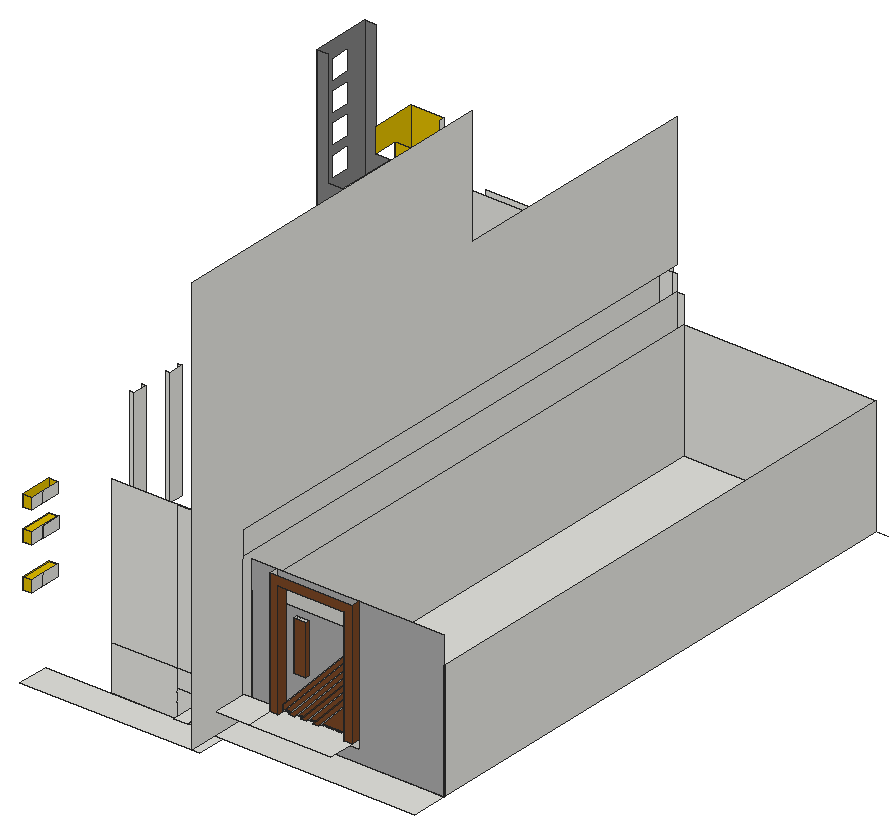
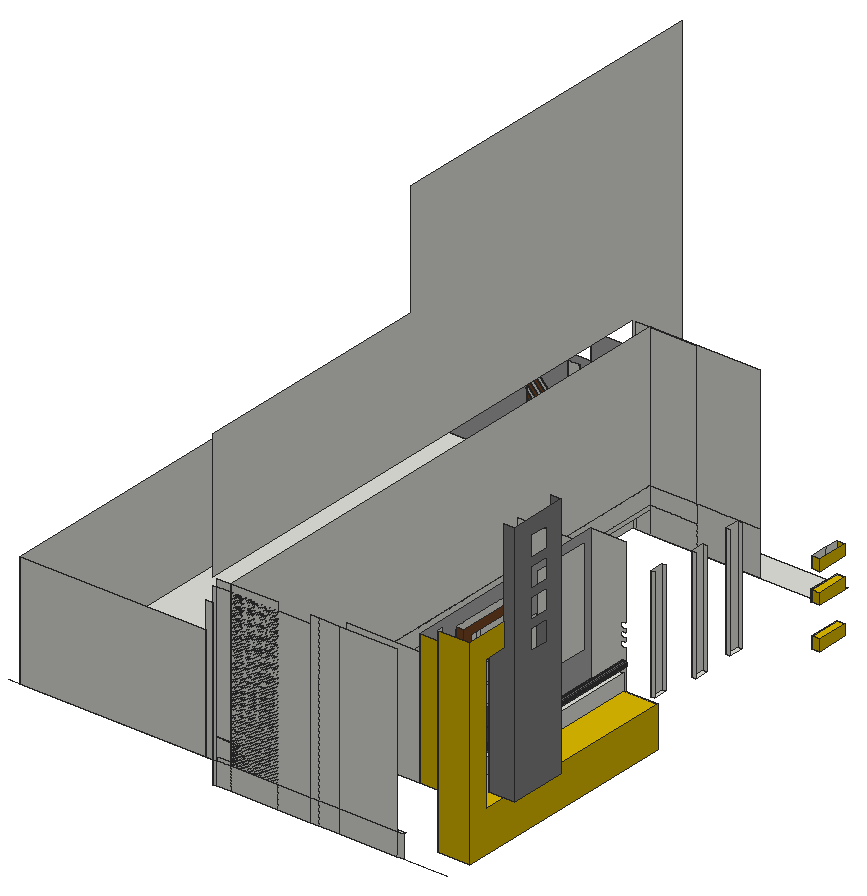
# SketchUp Ruby script. Lengths in inches.
U = 1.inch
M = Sketchup.active_model
def pt(a) = Geom::Point3d.new(a.map { |v| v * U })
def face(e, loops, mat)
  f = e.add_face(loops[0].map { |a| pt(a) })
  loops[1..].each { |l| e.add_face(l.map { |a| pt(a) }).erase! }
  f.material = f.back_material = mat if mat
  f
end
# faces: each face lists its corners as indices into pts; further lists are holes
def faces(e, pts, list, mat = nil) = list.each { |f| face(e, (f[0].is_a?(Array) ? f : [f]).map { |l| l.map { |i| pts[i] } }, mat) }
# xy, xz, yz: faces in a plane at the given z, y or x. An outline is a flat list of corners, or four numbers for a rectangle; further outlines are holes
def ring(l) = l.size == 4 ? [[l[0], l[1]], [l[2], l[1]], [l[2], l[3]], [l[0], l[3]]] : l.each_slice(2).to_a
def flat(e, list, mat, &to3) = list.each { |f| face(e, (f[0].is_a?(Array) ? f : [f]).map { |l| ring(l).map { |u, v| to3.(u, v) } }, mat) }
def xy(e, z, list, mat = nil) = flat(e, list, mat) { |x, y| [x, y, z] }
def xz(e, y, list, mat = nil) = flat(e, list, mat) { |x, z| [x, y, z] }
def yz(e, x, list, mat = nil) = flat(e, list, mat) { |y, z| [x, y, z] }
def lines(e, pts, list) = list.each { |a, b| e.add_line(pt(pts[a]), pt(pts[b])) }
# prism: a flat outline (further loops are holes) pulled along v
def prism(e, loops, v, mat = nil)
  f = face(e, loops, mat); d = Geom::Vector3d.new(v.map { |x| x * U })
  f.pushpull(f.normal.samedirection?(d) ? d.length : -d.length)
end
def box(e, o, s, mat = nil) = prism(e, [[o, [o[0] + s[0], o[1], o[2]], [o[0] + s[0], o[1] + s[1], o[2]], [o[0], o[1] + s[1], o[2]]]], [0, 0, s[2]], mat)
def at(x, y, z, deg = 0) = Geom::Transformation.translation(pt([x, y, z])) * Geom::Transformation.rotation(ORIGIN, Z_AXIS, deg.degrees)
def axes(o, x, y, z) = Geom::Transformation.new([*x, 0, *y, 0, *z, 0, *pt(o).to_a, 1])
def part(name) = M.definitions.add(name)
# library, detail: a bought-in or finely detailed component or shape, given as its bounding box
def library(name, o, s) = part(name).tap { |d| box(d.entities, o, s) }
def detail(e, o, s) = box(e.add_group.entities, o, s)
def put(e, d, t, mat = nil) = e.add_instance(d, t).tap { |i| i.material = mat if mat }
def group(e, t, mat = nil) = e.add_group.tap { |g| g.transformation = t; g.material = mat if mat }.entities
root = M.entities
M.materials.add("[0046_Gold]").color = [221, 186, 0]
M.materials.add("[0132_LightGray]").color = [169, 169, 169]
M.materials.add("[0133_Gray]").color = [128, 128, 128]
M.materials.add("[Wood Veneer 01]").color = [120, 70, 37]
xy(root,103.1875,[[138.64,72.5,269.16,95.5]])
xy(root,109.39,[[103,340.7,106,360.25],[103,363.42,106,386.14]])
xy(root,110.0625,[[100,416.8,103,466.49]],"[Wood Veneer 01]")
xy(root,112.39,[[103,337.7,106,389.14]])
xy(root,116.0625,[[100,410.8,106,472.49]],"[Wood Veneer 01]")
xy(root,117.15,[[88,138.31,94,162.08]],"[0046_Gold]")
xy(root,120,[[269.16,70.06,279.43,489.31],[279.43,70.06,279.47,489.31],[282.09,70.06,282.09,489.31,287.5,489.31,287.5,96.62,427.31,96.62,427.31,70.06],[287.5,96.62,427.31,489.31],[138.64,487.37,186.6,489.31]])
xy(root,123,[[269.16,95.5,279.43,489.31],[279.43,95.5,279.47,489.31]])
xy(root,123.47,[[82,479.49,106,494.21],[82,494.21,106,498.31]])
xy(root,123.47,[[82,322.08,106,479.49]],"[0046_Gold]")
xy(root,125.43,[[88,138.31,94,162.08]],"[0046_Gold]")
xy(root,133.96,[[106,245.52,109,256.27]])
xy(root,134.96,[[106,212.89,109,223.64]])
xy(root,136,[[269.16,49.06,279.43,489.31],[279.43,61.06,279.47,489.31]])
xy(root,136.21,[[279.47,70.06,306.51,95.5],[306.51,70.06,366.51,70.06,366.51,89.5,360.51,89.5,360.51,95.5,339.02,95.5,339.02,93.62,334.65,93.62,334.65,95.5,330.28,95.5,330.28,93.62,325.91,93.62,325.91,95.5,321.53,95.5,321.53,93.62,317.16,93.62,317.16,95.5,312.51,95.5,312.51,89.5,306.51,89.5],[306.51,89.5,312.51,95.5],[360.51,89.5,366.51,95.5],[317.16,93.62,321.53,95.5],
  [325.91,93.62,330.28,95.5],[334.65,93.62,339.02,95.5],[269.16,95.5,279.43,489.31],[279.43,95.5,279.47,489.31],[312.51,95.5,317.16,96.62],
  [317.16,95.5,321.53,96.62],[321.53,95.5,325.91,96.62],[325.91,95.5,330.28,96.62],[330.28,95.5,334.65,96.62],[334.65,95.5,339.02,96.62],
  [339.02,95.5,360.51,96.62]])
xy(root,137.52,[[106,283.77,109,294.52]])
xy(root,148.59,[[94,148.68,94.68,162.08]])
xy(root,148.59,[[88,138.31,94,162.08]],"[0046_Gold]")
xy(root,154.22,[[106.89,322.08,112.97,483.47],[112.97,322.08,131.78,322.08,131.78,388.87,125.78,388.87,125.78,394.87,128.78,394.87,128.78,442.87,125.78,442.87,125.78,448.87,131.78,448.87,131.78,483.47,112.97,483.47],[131.78,322.08,186.6,483.47],[125.78,388.87,131.78,394.87],[128.78,394.87,131.78,442.87],
  [73.87,422.6,82,466.21],[82,422.6,93.12,466.21],[125.78,442.87,131.78,448.87]])
xy(root,154.22,[[82,322.08,106.89,322.08,106.89,483.47,82,483.47,82,466.21,93.12,466.21,93.12,422.6,82,422.6]],"[0046_Gold]")
xy(root,156.87,[[94,148.68,94.68,162.08]])
xy(root,156.87,[[88,138.31,94,162.08]],"[0046_Gold]")
xy(root,164.28,[[320.34,93.62,329.34,96.62]])
xy(root,166.22,[[106.89,322.08,112.97,483.47]])
xy(root,171.09,[[88,138.31,94,162.08]],"[0046_Gold]")
xz(root,89.5,[[306.51,136.21,312.51,136.21,312.51,220.21,360.51,220.21,360.51,136.21,366.51,136.21,366.51,226.21,306.51,226.21]],"[Wood Veneer 01]")
xz(root,93.62,[[312.51,136.21,360.51,187.33,360.51,191.96,312.51,140.84],[317.16,136.21,321.53,136.21,360.51,177.72,360.51,182.38],[325.91,136.21,330.28,136.21,360.51,168.41,360.51,173.07],[334.65,136.21,339.02,136.21,360.51,159.1,360.51,163.75],[320.34,164.28,329.34,199.84]],"[Wood Veneer 01]")
xz(root,95.5,[[186.6,103.1875,233.78,136.21],[233.78,103.1875,269.16,123],[269.16,103.1875,279.43,123],[279.43,103.1875,282.09,123],[233.78,123,269.16,136.21],
  [269.16,123,279.43,136.21],[279.43,123,282.09,136.21],[306.51,130.21,366.51,136.21],[186.6,136.21,186.6,243,269.16,243,269.16,242.875,233.78,242.875,233.78,136.21],[233.78,136.21,269.16,242.875],
  [269.16,136.21,279.43,242.875],[279.43,136.21,282.09,225.3125]])
xz(root,96.62,[[427.31,120,427.68,205.375],[312.51,136.21,360.51,187.33,360.51,191.96,312.51,140.84],[317.16,136.21,321.53,136.21,360.51,177.72,360.51,182.38],[325.91,136.21,330.28,136.21,360.51,168.41,360.51,173.07],[334.65,136.21,339.02,136.21,360.51,159.1,360.51,163.75],
  [320.34,164.28,329.34,199.84]])
xz(root,96.62,[[[287.5,120,427.31,120,427.31,225.3125,287.5,225.3125,287.5,205.375,312.51,205.375,312.51,220.21,360.51,220.21,360.51,205.375,287.5,205.375],[312.51,136.21,312.51,140.84,360.51,191.96,360.51,136.21],[320.34,164.28,329.34,199.84]]],"[0132_LightGray]")
xz(root,96.62,[[312.51,136.21,317.16,136.21,360.51,182.38,360.51,187.33],[321.53,136.21,325.91,136.21,360.51,173.07,360.51,177.72],[330.28,136.21,334.65,136.21,360.51,163.75,360.51,168.41],[339.02,136.21,360.51,136.21,360.51,159.1]],"[Wood Veneer 01]")
xz(root,138.31,[[88,117.15,94,125.43],[88,148.59,94,156.87],[88,171.09,94,179.37]],"[0046_Gold]")
xz(root,148.68,[[94,148.59,94.68,156.87]])
xz(root,162.08,[[94,148.59,94.68,156.87]])
xz(root,162.08,[[88,117.15,94,125.43],[88,148.59,94,156.87],[88,171.09,94,179.37]],"[0046_Gold]")
xz(root,212.89,[[106,134.96,109,219.9]])
xz(root,223.64,[[106,134.96,109,219.9]])
xz(root,245.52,[[106,133.96,109,218.9]])
xz(root,256.27,[[106,133.96,109,218.9]])
xz(root,283.77,[[106,137.52,109,222.46]])
xz(root,294.52,[[106,137.52,109,222.46]])
xz(root,322.08,[[106,154.22,106,170.63,106.12,170.54,106.66,170.32,107.24,170.24,107.82,170.32,108.37,170.54,108.83,170.9,109.1875,171.36,109.41,171.91,109.49,172.49,109.41,173.07,109.1875,173.61,108.83,174.08,108.37,174.4375,107.82,174.66,107.24,174.74,106.66,174.66,106.12,174.4375,106,174.35,106,183.63,106.12,183.54,106.66,183.32,107.24,183.24,107.82,183.32,108.37,183.54,108.83,183.9,109.1875,184.36,109.41,184.91,109.49,185.49,109.41,186.07,109.1875,186.61,108.83,187.08,108.37,187.4375,107.82,187.66,107.24,187.74,106.66,187.66,106.12,187.4375,106,187.35,106,190.13,106.12,190.04,106.66,189.82,107.24,189.74,107.82,189.82,108.37,190.04,108.83,190.4,109.1875,190.86,109.41,191.41,109.49,191.99,109.41,192.57,109.1875,193.11,108.83,193.58,108.37,193.9375,107.82,194.16,107.24,194.24,106.66,194.16,106.12,193.9375,106,193.85,106,196.63,106.12,196.54,106.66,196.32,107.24,196.24,107.82,196.32,108.37,196.54,108.83,196.9,109.1875,197.36,109.41,197.91,109.49,198.49,109.41,199.07,109.1875,199.61,108.83,200.08,108.37,200.4375,107.82,200.66,107.24,200.74,106.66,200.66,106.12,200.4375,106,200.35,106,255.04,131.78,255.04,131.78,154.22,112.97,154.22,112.97,166.22,106.89,166.22,106.89,154.22],[106.89,154.22,112.97,166.22],[131.78,154.22,186.6,243],[107.24,170.24,107.82,170.32,108.37,170.54,108.83,170.9,109.1875,171.36,109.41,171.91,109.49,172.49,109.41,173.07,109.1875,173.61,108.83,174.08,108.37,174.4375,107.82,174.66,107.24,174.74,106.66,174.66,106.12,174.4375,106,174.35,106,170.63,106.12,170.54,106.66,170.32],[106,170.63,106,174.35,105.65,174.08,105.29,173.61,105.07,173.07,104.99,172.49,105.07,171.91,105.29,171.36,105.65,170.9]])
xz(root,322.08,[[82,123.47,106,154.22]],"[0046_Gold]")
xz(root,388.87,[[125.78,154.22,131.78,244.22]],"[Wood Veneer 01]")
xz(root,394.87,[[128.78,154.22,131.78,238.22]])
xz(root,394.87,[[125.78,154.22,128.78,238.22]],"[Wood Veneer 01]")
xz(root,422.6,[[73.87,154.22,93.12,154.22,93.12,255.04,82,255.04,82,339,73.87,339]],"[0133_Gray]")
xz(root,442.87,[[128.78,154.22,131.78,238.22]])
xz(root,442.87,[[125.78,154.22,128.78,238.22]],"[Wood Veneer 01]")
xz(root,448.87,[[125.78,154.22,131.78,244.22]],"[Wood Veneer 01]")
xz(root,466.21,[[73.87,154.22,73.87,339,82,339,82,255.04,93.12,255.04,93.12,154.22]],"[0133_Gray]")
xz(root,483.47,[[106.89,154.22,112.97,166.22],[131.78,154.22,186.6,243]])
xz(root,483.47,[[[82,154.22,106.89,154.22,106.89,166.22,112.97,166.22,112.97,154.22,131.78,154.22,131.78,255.04,82,255.04],[107.24,170.24,106.66,170.32,106.12,170.54,105.65,170.9,105.29,171.36,105.07,171.91,104.99,172.49,105.07,173.07,105.29,173.61,105.65,174.08,106.12,174.4375,106.66,174.66,107.24,174.74,107.82,174.66,108.37,174.4375,108.83,174.08,109.1875,173.61,109.41,173.07,109.49,172.49,109.41,171.91,109.1875,171.36,108.83,170.9,108.37,170.54,107.82,170.32],[107.24,176.74,106.66,176.82,106.12,177.04,105.65,177.4,105.29,177.86,105.07,178.41,104.99,178.99,105.07,179.57,105.29,180.11,105.65,180.58,106.12,180.9375,106.66,181.16,107.24,181.24,107.82,181.16,108.37,180.9375,108.83,180.58,109.1875,180.11,109.41,179.57,109.49,178.99,109.41,178.41,109.1875,177.86,108.83,177.4,108.37,177.04,107.82,176.82],[107.24,183.24,106.66,183.32,106.12,183.54,105.65,183.9,105.29,184.36,105.07,184.91,104.99,185.49,105.07,186.07,105.29,186.61,105.65,187.08,106.12,187.4375,106.66,187.66,107.24,187.74,107.82,187.66,108.37,187.4375,108.83,187.08,109.1875,186.61,109.41,186.07,109.49,185.49,109.41,184.91,109.1875,184.36,108.83,183.9,108.37,183.54,107.82,183.32],[107.24,189.74,106.66,189.82,106.12,190.04,105.65,190.4,105.29,190.86,105.07,191.41,104.99,191.99,105.07,192.57,105.29,193.11,105.65,193.58,106.12,193.9375,106.66,194.16,107.24,194.24,107.82,194.16,108.37,193.9375,108.83,193.58,109.1875,193.11,109.41,192.57,109.49,191.99,109.41,191.41,109.1875,190.86,108.83,190.4,108.37,190.04,107.82,189.82],[107.24,196.24,106.66,196.32,106.12,196.54,105.65,196.9,105.29,197.36,105.07,197.91,104.99,198.49,105.07,199.07,105.29,199.61,105.65,200.08,106.12,200.4375,106.66,200.66,107.24,200.74,107.82,200.66,108.37,200.4375,108.83,200.08,109.1875,199.61,109.41,199.07,109.49,198.49,109.41,197.91,109.1875,197.36,108.83,196.9,108.37,196.54,107.82,196.32]]],"[0046_Gold]")
xz(root,489.31,[[138.64,103.1875,143.81,120],[143.81,103.1875,186.6,120],[186.6,103.1875,202.62,120],[202.62,103.1875,208.53,120],[208.53,103.1875,233.78,120],
  [233.78,103.1875,269.16,120],[269.16,103.1875,279.43,120],[279.43,103.1875,282.09,120],[143.81,120,186.6,243],[186.6,120,202.62,243],
  [202.62,120,208.53,243],[208.53,120,208.53,237.125,233.78,237.125,233.78,242.875,279.43,242.875,279.43,237.125,269.16,237.125,269.16,120],[208.53,120,233.78,237.125],[233.78,120,269.16,237.125],[269.16,120,279.43,123],
  [279.43,120,279.47,123],[279.47,120,279.47,123,279.43,123,279.43,136,279.47,136,279.47,136.21,279.43,136.21,279.43,237.125,282.09,237.125,282.09,120],[282.09,120,287.5,225.3125],[287.5,120,427.31,205.375],[269.16,123,279.43,136],
  [269.16,136,279.43,136.21],[279.43,136,279.47,136.21],[269.16,136.21,279.43,237.125]])
xz(root,498.31,[[82,123.47,106,272.6]],"[0046_Gold]")
yz(root,73.87,[[[422.6,154.22,466.21,339],[436.12,312.39,451.12,327.39],[436.12,291.33,451.12,306.33],[436.12,270.27,451.12,285.27],[436.12,249.21,451.12,264.21]]],"[0133_Gray]")
yz(root,82,[[322.08,123.47,322.08,154.22,483.47,154.22,483.47,255.04,466.21,255.04,466.21,272.6,498.31,272.6,498.31,123.47]],"[0046_Gold]")
yz(root,88,[[138.31,117.15,162.08,125.43],[138.31,148.59,162.08,156.87],[138.31,171.09,162.08,179.37]],"[0046_Gold]")
yz(root,93.12,[[422.6,154.22,466.21,255.04]])
yz(root,94,[[138.31,117.15,148.68,125.43],[148.68,117.15,162.08,125.43],[138.31,148.59,148.68,156.87],[148.68,148.59,162.08,156.87],[138.31,171.09,148.68,179.37],
  [148.68,171.09,162.08,179.37]])
yz(root,94.68,[[148.68,148.59,162.08,156.87]])
yz(root,106,[[494.21,123.47,498.31,272.6]])
yz(root,106.89,[[322.08,154.22,483.47,166.22]])
yz(root,109,[[245.52,133.96,256.27,218.9],[212.89,134.96,223.64,219.9],[283.77,137.52,294.52,222.46]])
yz(root,112.97,[[322.08,154.22,483.47,166.22]])
yz(root,125.78,[[388.87,154.22,388.87,244.22,448.87,244.22,448.87,154.22,442.87,154.22,442.87,238.22,394.87,238.22,394.87,154.22]],"[Wood Veneer 01]")
yz(root,128.78,[[430.4,154.22,430.4,166.08,394.87,166.08,394.87,167.22,430.4,167.22,430.4,180.96,394.87,180.96,394.87,182.1,430.4,182.1,430.4,195.83,394.87,195.83,394.87,196.97,430.4,196.97,430.4,210.71,394.87,210.71,394.87,211.85,430.4,211.85,430.4,225.58,394.87,225.58,394.87,226.72,430.4,226.72,430.4,238.22,433.39,238.22,433.39,226.72,442.87,226.72,442.87,225.58,433.39,225.58,433.39,211.85,442.87,211.85,442.87,210.71,433.39,210.71,433.39,196.97,442.87,196.97,442.87,195.83,433.39,195.83,433.39,182.1,442.87,182.1,442.87,180.96,433.39,180.96,433.39,167.22,442.87,167.22,442.87,166.08,433.39,166.08,433.39,154.22]])
yz(root,128.78,[[394.87,154.22,430.4,166.08],[433.39,154.22,442.87,166.08],[394.87,167.22,430.4,180.96],[433.39,167.22,442.87,180.96]],"[Wood Veneer 01]")
yz(root,131.78,[[388.87,148.22,448.87,154.22],[388.87,154.22,394.87,154.22,394.87,238.22,442.87,238.22,442.87,154.22,448.87,154.22,448.87,244.22,388.87,244.22],[394.87,154.22,442.87,238.22]])
yz(root,131.78,[[[322.08,154.22,322.08,255.04,483.47,255.04,483.47,154.22,448.87,154.22,448.87,244.22,388.87,244.22,388.87,154.22],[328.14,175.8125,373.08,248.52]]],"[0132_LightGray]")
yz(root,269.16,[[95.5,120,489.31,123],[95.5,123,489.31,136],[95.5,136,489.31,136.21],[95.5,136.21,489.31,242.875]])
yz(root,279.47,[[61.06,120,489.31,123],[49.06,136,489.31,136.21]])
yz(root,282.09,[[95.5,103.1875,489.31,120],[49.06,120,95.5,120,95.5,242.875,489.31,242.875,489.31,339,303.56,339,303.56,424.32,49.06,424.32],[95.5,120,489.31,225.3125]])
yz(root,287.5,[[96.62,120,489.31,205.375]])
yz(root,306.51,[[89.5,136.21,95.5,226.21]])
yz(root,312.51,[[93.62,136.21,96.62,140.84]])
yz(root,312.51,[[89.5,136.21,93.62,136.21,93.62,140.84,96.62,140.84,96.62,220.21,89.5,220.21]],"[Wood Veneer 01]")
yz(root,320.34,[[93.62,164.28,96.62,199.84]])
yz(root,329.34,[[93.62,164.28,96.62,199.84]],"[Wood Veneer 01]")
yz(root,360.51,[[93.62,159.1,96.62,163.75],[93.62,168.41,96.62,173.07]])
yz(root,360.51,[[89.5,136.21,89.5,220.21,96.62,220.21,96.62,191.96,93.62,191.96,93.62,187.33,96.62,187.33,96.62,182.38,93.62,182.38,93.62,177.72,96.62,177.72,96.62,173.07,93.62,173.07,93.62,168.41,96.62,168.41,96.62,163.75,93.62,163.75,93.62,159.1,96.62,159.1,96.62,136.21]],"[Wood Veneer 01]")
yz(root,366.51,[[89.5,136.21,95.5,226.21]],"[Wood Veneer 01]")
yz(root,427.31,[[96.62,120,489.31,205.375]])
p = [[312.51,96.62,136.21],[360.51,96.62,187.33],[360.51,93.62,187.33],[312.51,93.62,136.21],[312.51,95.5,136.21],[360.51,96.62,182.38],
  [317.16,96.62,136.21],[317.16,95.5,136.21],[317.16,93.62,136.21],[360.51,93.62,182.38],[321.53,96.62,136.21],[360.51,96.62,177.72],
  [360.51,93.62,177.72],[321.53,93.62,136.21],[321.53,95.5,136.21],[360.51,96.62,173.07],[325.91,96.62,136.21],[325.91,95.5,136.21],
  [325.91,93.62,136.21],[360.51,93.62,173.07],[330.28,96.62,136.21],[360.51,96.62,168.41],[360.51,93.62,168.41],[330.28,93.62,136.21],
  [330.28,95.5,136.21],[360.51,96.62,163.75],[334.65,96.62,136.21],[334.65,95.5,136.21],[334.65,93.62,136.21],[360.51,93.62,163.75],
  [339.02,96.62,136.21],[360.51,96.62,159.1],[360.51,93.62,159.1],[339.02,93.62,136.21],[339.02,95.5,136.21],[360.51,96.62,191.96],
  [312.51,96.62,140.84],[312.51,93.62,140.84],[360.51,93.62,191.96],[106.66,483.47,170.32],[107.24,483.47,170.24],[107.24,322.08,170.24],
  [106.66,322.08,170.32],[107.82,483.47,170.32],[107.82,322.08,170.32],[106.12,483.47,170.54],[106.12,322.08,170.54],[108.37,483.47,170.54],
  [108.37,322.08,170.54],[105.65,483.47,170.9],[106,322.08,170.63],[105.65,322.08,170.9],[108.83,483.47,170.9],[108.83,322.08,170.9],
  [105.29,483.47,171.36],[105.29,322.08,171.36],[109.1875,483.47,171.36],[109.1875,322.08,171.36],[105.07,483.47,171.91],[105.07,322.08,171.91],
  [109.41,483.47,171.91],[109.41,322.08,171.91],[104.99,483.47,172.49],[104.99,322.08,172.49],[109.49,483.47,172.49],[109.49,322.08,172.49],
  [105.07,483.47,173.07],[105.07,322.08,173.07],[109.41,483.47,173.07],[109.41,322.08,173.07],[105.29,483.47,173.61],[105.29,322.08,173.61],
  [109.1875,483.47,173.61],[109.1875,322.08,173.61],[105.65,483.47,174.08],[105.65,322.08,174.08],[108.83,483.47,174.08],[108.83,322.08,174.08],
  [106.12,483.47,174.4375],[106,322.08,174.35],[106.12,322.08,174.4375],[108.37,483.47,174.4375],[108.37,322.08,174.4375],[106.66,483.47,174.66],
  [106.66,322.08,174.66],[107.82,483.47,174.66],[107.82,322.08,174.66],[107.24,483.47,174.74],[107.24,322.08,174.74],[316.17,96.62,135.16],
  [317.88,96.62,132.32],[318.87,96.62,133.37],[319.58,96.62,129.48],[320.57,96.62,130.53],[363.92,96.62,176.7],[321.29,96.62,126.64],
  [322.28,96.62,127.69],[365.625,96.62,173.86],[322.99,96.62,123.8],[323.98,96.62,124.85],[324.7,96.62,120.96],[325.6875,96.62,122.01],
  [427.31,489.31,120],[436.31,489.31,120],[106,489.31,103.1875],[138.64,489.31,103.1875]]
faces(root,p,[[0,1,2,3,4],[5,6,7,8,9],[10,11,12,13,14],[20,21,22,23,24],[30,31,32,33,34],[35,36,37,38]])
faces(root,p,[[15,16,17,18,19],[25,26,27,28,29]],"[Wood Veneer 01]")
faces(root,p,[[39,40,41,42],[40,43,44,41],[45,39,42,46],[43,47,48,44],[49,45,46,50,51],[47,52,53,48],[54,49,51,55],[52,56,57,53],
  [58,54,55,59],[56,60,61,57],[62,58,59,63],[60,64,65,61],[66,62,63,67],[64,68,69,65],[70,66,67,71],[68,72,73,69],
  [74,70,71,75],[72,76,77,73],[78,74,75,79,80],[76,81,82,77],[83,78,80,84],[81,85,86,82],[87,83,84,88],[85,87,88,86]],"[0133_Gray]")
lines(root,p,[[89,6],[90,91],[91,10],[92,93],[93,16],[15,94],[95,96],[96,20],[21,97],[98,99],[99,26],[100,101],
  [101,30],[102,103],[104,105]])
